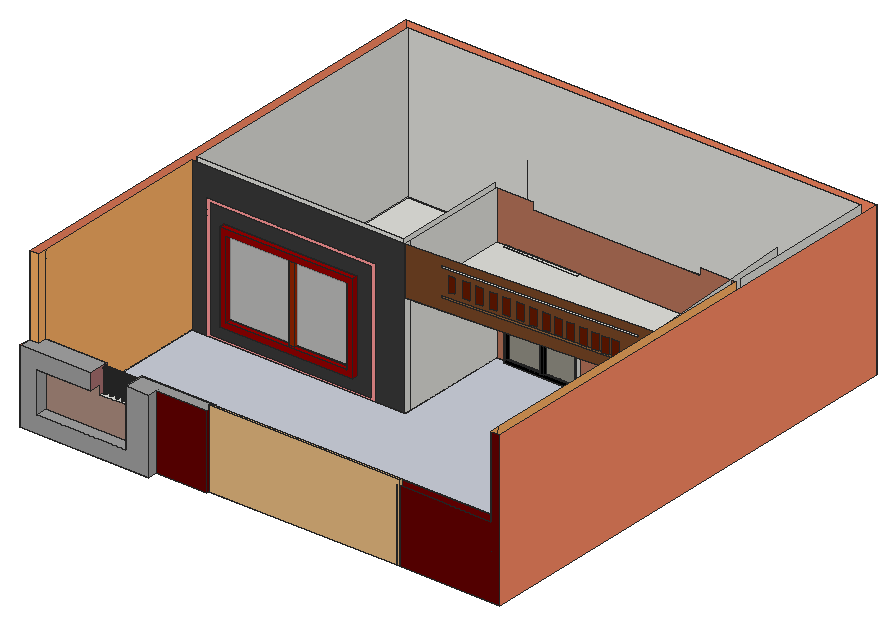
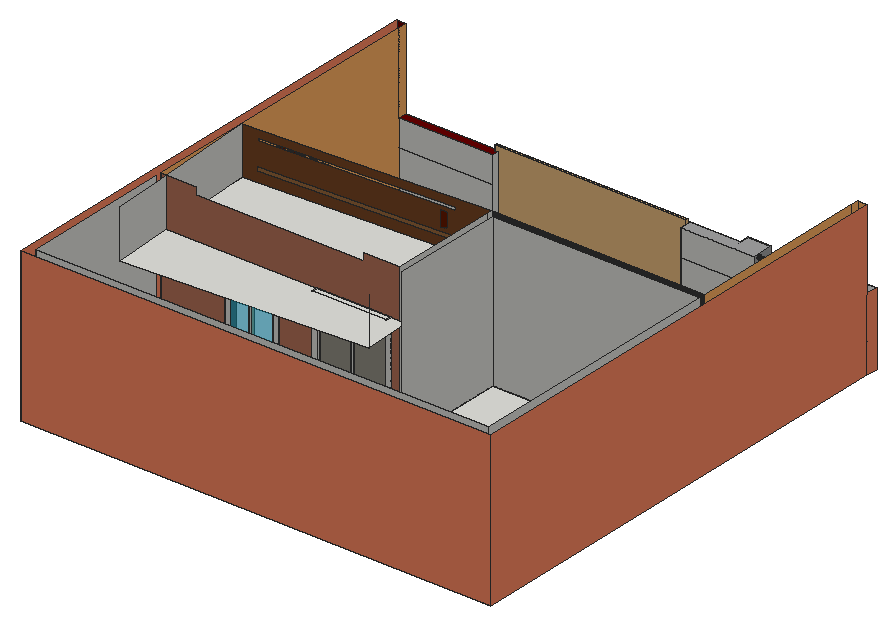
# SketchUp Ruby script. Lengths in inches.
U = 1.inch
M = Sketchup.active_model
def pt(a) = Geom::Point3d.new(a.map { |v| v * U })
def face(e, loops, mat)
  f = e.add_face(loops[0].map { |a| pt(a) })
  loops[1..].each { |l| e.add_face(l.map { |a| pt(a) }).erase! }
  f.material = f.back_material = mat if mat
  f
end
# faces: each face lists its corners as indices into pts; further lists are holes
def faces(e, pts, list, mat = nil) = list.each { |f| face(e, (f[0].is_a?(Array) ? f : [f]).map { |l| l.map { |i| pts[i] } }, mat) }
# xy, xz, yz: faces in a plane at the given z, y or x. An outline is a flat list of corners, or four numbers for a rectangle; further outlines are holes
def ring(l) = l.size == 4 ? [[l[0], l[1]], [l[2], l[1]], [l[2], l[3]], [l[0], l[3]]] : l.each_slice(2).to_a
def flat(e, list, mat, &to3) = list.each { |f| face(e, (f[0].is_a?(Array) ? f : [f]).map { |l| ring(l).map { |u, v| to3.(u, v) } }, mat) }
def xy(e, z, list, mat = nil) = flat(e, list, mat) { |x, y| [x, y, z] }
def xz(e, y, list, mat = nil) = flat(e, list, mat) { |x, z| [x, y, z] }
def yz(e, x, list, mat = nil) = flat(e, list, mat) { |y, z| [x, y, z] }
def lines(e, pts, list) = list.each { |a, b| e.add_line(pt(pts[a]), pt(pts[b])) }
# prism: a flat outline (further loops are holes) pulled along v
def prism(e, loops, v, mat = nil)
  f = face(e, loops, mat); d = Geom::Vector3d.new(v.map { |x| x * U })
  f.pushpull(f.normal.samedirection?(d) ? d.length : -d.length)
end
def box(e, o, s, mat = nil) = prism(e, [[o, [o[0] + s[0], o[1], o[2]], [o[0] + s[0], o[1] + s[1], o[2]], [o[0], o[1] + s[1], o[2]]]], [0, 0, s[2]], mat)
def at(x, y, z, deg = 0) = Geom::Transformation.translation(pt([x, y, z])) * Geom::Transformation.rotation(ORIGIN, Z_AXIS, deg.degrees)
def axes(o, x, y, z) = Geom::Transformation.new([*x, 0, *y, 0, *z, 0, *pt(o).to_a, 1])
def part(name) = M.definitions.add(name)
# library, detail: a bought-in or finely detailed component or shape, given as its bounding box
def library(name, o, s) = part(name).tap { |d| box(d.entities, o, s) }
def detail(e, o, s) = box(e.add_group.entities, o, s)
def put(e, d, t, mat = nil) = e.add_instance(d, t).tap { |i| i.material = mat if mat }
def group(e, t, mat = nil) = e.add_group.tap { |g| g.transformation = t; g.material = mat if mat }.entities
root = M.entities
M.materials.add("[Color A02]").color = [255, 153, 153]
M.materials.add("[Color A07]").color = [153, 0, 0]
M.materials.add("[Color A08]").color = [102, 0, 0]
M.materials.add("[Color B03]").color = [255, 140, 101]
M.materials.add("[Color B07]").color = [153, 38, 0]
M.materials.add("[Color B08]").color = [102, 25, 0]
M.materials.add("[Color C03]").color = [255, 178, 101]
M.materials.add("[Color M06]").color = [86, 86, 86]
M.materials.add("[Color M07]").color = [58, 58, 58]
M.materials.add("[Color M09]").color = [0, 0, 0]
M.materials.add("[Formica Beige]").color = [211, 187, 149]
M.materials.add("[Formica Graystone]").color = [149, 146, 135]
M.materials.add("[Formica Speckled Grey]").color = [94, 105, 111]
M.materials.add("[Marble Carrara Floor Tile]").color = [204, 208, 219]
M.materials.add("[Metal Rusted]").color = [184, 117, 91]
M.materials.add("[Pavers Flagstone Gray]").color = [162, 162, 162]
M.materials.add("[Pavers Herringbone Brick]").color = [172, 115, 115]
M.materials.add("[Pavers Modular Brick]").color = [175, 143, 129]
M.materials.add("[Translucent Glass Tinted]").color = [8, 201, 241]
M.materials["[Translucent Glass Tinted]"].alpha = 0.48
M.materials.add("[Translucent Resin Crush Gray]").color = [184, 184, 184]
M.materials["[Translucent Resin Crush Gray]"].alpha = 0.8
M.materials.add("[Wood Floor]").color = [155, 105, 61]
M.materials.add("[Wood Veneer 01]").color = [120, 70, 37]
c1 = library("Modern+Gate+1",[0,0,0],[118.11,1.97,78.74])
xy(root,0,[[1.5,7.75,132.625,19.75],[132.625,16.75,132.625,19.75,1.5,19.75,1.5,499.75,481.5,499.75,481.5,19.75,376.06,19.75,376.06,28.75,472.5,28.75,472.5,331.6875,313.15,331.6875,313.15,337.6875,472.5,337.6875,472.5,490.75,10.5,490.75,10.5,221.25,222.3125,221.25,222.3125,337.6875,237.6875,337.6875,237.6875,331.6875,228.3125,331.6875,228.3125,215.25,10.5,215.25,10.5,28.75,184.33,28.75,184.33,16.75],[10.5,28.75,10.5,215.25,228.3125,215.25,228.3125,331.6875,237.6875,331.6875,237.6875,337.6875,313.15,337.6875,313.15,331.6875,472.5,331.6875,472.5,28.75],[10.5,221.25,10.5,490.75,472.5,490.75,472.5,337.6875,222.3125,337.6875,222.3125,221.25]])
xy(root,1.0625,[[237.6875,328.6875,313.15,331.6875],[237.6875,331.6875,313.15,337.6875]])
xy(root,1.0625,[[10.5,28.75,472.5,28.75,472.5,331.6875,313.15,331.6875,313.15,328.6875,237.6875,328.6875,237.6875,331.6875,228.3125,331.6875,228.3125,215.25,10.5,215.25]],"[Marble Carrara Floor Tile]")
xy(root,1.125,[[10.5,221.25,222.3125,221.25,222.3125,337.6875,472.5,337.6875,472.5,490.75,10.5,490.75]])
xy(root,4.0625,[[275.42,328.6875,279.09,331.6875]])
xy(root,4.0625,[[240.6875,328.6875,275.42,331.6875],[279.09,328.6875,310.15,331.6875]],"[Color M09]")
xy(root,17.12,[[18.4,7.75,108.71,19.75]],"[Pavers Flagstone Gray]")
xy(root,17.84,[[43.625,209.25,179.38,215.25]],"[Color A07]")
xy(root,23.84,[[111.5,212.25,117.62,215.25]])
xy(root,23.84,[[49.625,209.25,173.38,209.25,173.38,215.25,117.62,215.25,117.62,212.25,111.5,212.25,111.5,215.25,49.625,215.25]],"[Color A07]")
xy(root,26.73,[[352.36,325.6875,407.17,331.6875]])
xy(root,32.73,[[379.77,328.6875,382.79,331.6875]])
xy(root,32.73,[[358.36,325.6875,401.17,325.6875,401.17,331.6875,382.79,331.6875,382.79,328.6875,379.77,328.6875,379.77,331.6875,358.36,331.6875]],"[Formica Speckled Grey]")
xy(root,49.75,[[[73.27,19.75,108.71,28.75],[75.43,22.84,74.98,22.89,74.55,23.0625,74.1875,23.33,73.9,23.69,73.72,24.11,73.65,24.5625,73.7,25.02,73.87,25.44,74.14,25.81,74.5,26.09,74.92,26.28,75.37,26.34,75.82,26.29,76.25,26.125,76.62,25.85,76.9,25.5,77.08,25.08,77.15,24.625,77.1,24.17,76.93,23.75,76.66,23.38,76.3,23.09,75.89,22.91],[81.31,22.84,80.85,22.89,80.43,23.0625,80.0625,23.33,79.78,23.69,79.6,24.11,79.53,24.5625,79.58,25.02,79.75,25.44,80.02,25.81,80.375,26.09,80.79,26.28,81.24,26.34,81.7,26.29,82.125,26.125,82.49,25.85,82.78,25.5,82.96,25.08,83.03,24.625,82.98,24.17,82.81,23.75,82.54,23.38,82.18,23.09,81.76,22.91],[87.31,22.84,86.85,22.89,86.43,23.0625,86.0625,23.33,85.78,23.69,85.6,24.11,85.53,24.5625,85.58,25.02,85.75,25.44,86.02,25.81,86.375,26.09,86.79,26.28,87.24,26.34,87.7,26.29,88.125,26.125,88.49,25.85,88.78,25.5,88.96,25.08,89.03,24.625,88.98,24.17,88.81,23.75,88.54,23.38,88.18,23.09,87.76,22.91],[93.39,22.91,92.9375,22.96,92.51,23.125,92.15,23.4,91.86,23.75,91.68,24.17,91.61,24.625,91.66,25.08,91.83,25.5,92.1,25.87,92.46,26.15,92.88,26.34,93.33,26.41,93.78,26.35,94.21,26.1875,94.58,25.92,94.86,25.56,95.04,25.14,95.11,24.6875,95.06,24.23,94.89,23.81,94.62,23.44,94.26,23.16,93.84,22.97],[99.52,22.91,99.0625,22.96,98.64,23.125,98.27,23.4,97.99,23.75,97.8,24.17,97.74,24.625,97.79,25.08,97.95,25.5,98.23,25.87,98.58,26.15,99,26.34,99.45,26.41,99.91,26.35,100.33,26.1875,100.7,25.92,100.99,25.56,101.17,25.14,101.24,24.6875,101.18,24.23,101.02,23.81,100.75,23.44,100.39,23.16,99.97,22.97],[106.08,22.91,105.625,22.96,105.2,23.125,104.83,23.4,104.55,23.75,104.37,24.17,104.3,24.625,104.35,25.08,104.52,25.5,104.79,25.87,105.15,26.15,105.56,26.34,106.02,26.41,106.47,26.35,106.9,26.1875,107.26,25.92,107.55,25.56,107.73,25.14,107.8,24.6875,107.75,24.23,107.58,23.81,107.31,23.44,106.95,23.16,106.53,22.97]],[87.31,22.84,86.85,22.89,86.43,23.0625,86.0625,23.33,85.78,23.69,85.6,24.11,85.53,24.5625,85.58,25.02,85.75,25.44,86.02,25.81,86.375,26.09,86.79,26.28,87.24,26.34,87.7,26.29,88.125,26.125,88.49,25.85,88.78,25.5,88.96,25.08,89.03,24.625,88.98,24.17,88.81,23.75,88.54,23.38,88.18,23.09,87.76,22.91],[93.39,22.91,92.9375,22.96,92.51,23.125,92.15,23.4,91.86,23.75,91.68,24.17,91.61,24.625,91.66,25.08,91.83,25.5,92.1,25.87,92.46,26.15,92.88,26.34,93.33,26.41,93.78,26.35,94.21,26.1875,94.58,25.92,94.86,25.56,95.04,25.14,95.11,24.6875,95.06,24.23,94.89,23.81,94.62,23.44,94.26,23.16,93.84,22.97]])
xy(root,58.43,[[18.4,7.75,73.27,19.75]],"[Pavers Flagstone Gray]")
xy(root,71.625,[[81.31,22.84,81.76,22.91,82.18,23.09,82.54,23.38,82.81,23.75,82.97,24.16,82.98,24.17,83.03,24.625,82.96,25.08,82.78,25.5,82.65,25.66,82.49,25.85,82.125,26.125,81.7,26.29,81.24,26.34,80.79,26.28,80.375,26.09,80.02,25.81,79.91,25.66,79.75,25.44,79.58,25.02,79.53,24.5625,79.59,24.16,79.6,24.11,79.78,23.69,80.0625,23.33,80.43,23.0625,80.85,22.89]])
xy(root,71.86,[[87.31,22.84,87.76,22.91,88.18,23.09,88.54,23.38,88.81,23.75,88.85,23.85,85.71,23.85,85.78,23.69,86.0625,23.33,86.43,23.0625,86.85,22.89],[93.39,22.91,93.84,22.97,94.26,23.16,94.62,23.44,94.89,23.81,94.91,23.85,91.82,23.85,91.86,23.75,92.15,23.4,92.51,23.125,92.9375,22.96],[106.08,22.91,106.53,22.97,106.95,23.16,107.31,23.44,107.58,23.81,107.6,23.85,104.51,23.85,104.55,23.75,104.83,23.4,105.2,23.125,105.625,22.96],[85.71,23.85,88.85,23.85,88.98,24.17,89.03,24.625,88.96,25.08,88.78,25.5,88.49,25.85,88.34,25.97,86.22,25.97,86.02,25.81,85.75,25.44,85.58,25.02,85.53,24.5625,85.6,24.11],[91.82,23.85,94.91,23.85,95.06,24.23,95.11,24.6875,95.04,25.14,94.86,25.56,94.58,25.92,94.5,25.97,92.22,25.97,92.1,25.87,91.83,25.5,91.66,25.08,91.61,24.625,91.68,24.17],
  [104.51,23.85,107.6,23.85,107.75,24.23,107.8,24.6875,107.73,25.14,107.55,25.56,107.26,25.92,107.19,25.97,104.91,25.97,104.79,25.87,104.52,25.5,104.35,25.08,104.3,24.625,104.37,24.17],[86.22,25.97,88.34,25.97,88.125,26.125,87.7,26.29,87.24,26.34,86.79,26.28,86.375,26.09],[92.22,25.97,92.46,26.15,92.88,26.34,93.33,26.41,93.78,26.35,94.21,26.1875,94.5,25.97],[104.91,25.97,107.19,25.97,106.9,26.1875,106.47,26.35,106.02,26.41,105.56,26.34,105.15,26.15]])
xy(root,71.9375,[[75.43,22.84,75.89,22.91,76.3,23.09,76.66,23.38,76.93,23.75,77.1,24.17,77.15,24.625,77.08,25.08,76.9,25.5,76.62,25.85,76.25,26.125,75.82,26.29,75.37,26.34,74.92,26.28,74.5,26.09,74.14,25.81,73.87,25.44,73.7,25.02,73.65,24.5625,73.72,24.11,73.9,23.69,74.1875,23.33,74.55,23.0625,74.98,22.89]])
xy(root,72.17,[[99.52,22.91,99.97,22.97,100.39,23.16,100.75,23.44,100.87,23.61,98.1,23.61,98.27,23.4,98.64,23.125,99.0625,22.96],[98.1,23.61,100.87,23.61,101.02,23.81,101.18,24.23,101.24,24.6875,101.17,25.14,100.99,25.56,100.7,25.92,100.33,26.1875,100.28,26.21,98.7,26.21,98.58,26.15,98.23,25.87,97.95,25.5,97.79,25.08,97.74,24.625,97.8,24.17,97.99,23.75],[98.7,26.21,100.28,26.21,99.91,26.35,99.45,26.41,99,26.34]])
xy(root,73.875,[[376.06,19.75,472.5,28.75]],"[Color A08]")
xy(root,74.8125,[[1.5,7.75,73.27,7.75,73.27,28.75,10.5,28.75,10.5,19.75,1.5,19.75],[108.71,7.75,132.625,7.75,132.625,16.75,184.33,16.75,184.33,28.75,108.71,28.75]],"[Pavers Flagstone Gray]")
xy(root,83.04,[[379.77,328.6875,382.79,331.6875]])
xy(root,83.04,[[358.36,325.6875,358.36,331.6875,379.77,331.6875,379.77,328.6875,382.79,328.6875,382.79,331.6875,401.17,331.6875,401.17,325.6875]],"[Formica Speckled Grey]")
xy(root,89.04,[[352.36,325.6875,407.17,331.6875]],"[Formica Speckled Grey]")
xy(root,103.33,[[111.5,212.25,117.62,215.25]])
xy(root,103.33,[[49.625,209.25,49.625,215.25,111.5,215.25,111.5,212.25,117.62,212.25,117.62,215.25,173.38,215.25,173.38,209.25]],"[Color A07]")
xy(root,104.07,[[275.42,328.6875,279.09,331.6875]])
xy(root,104.07,[[240.6875,328.6875,275.42,331.6875],[279.09,328.6875,310.15,331.6875]],"[Color M09]")
xy(root,107.07,[[[228.3125,215.25,219.69,382.03,463.88,394.65,472.5,227.87],[237.6875,328.6875,313.15,337.6875]],[237.6875,328.6875,313.15,331.6875],[237.6875,331.6875,313.15,337.6875]])
xy(root,109.33,[[43.625,209.25,179.38,215.25]],"[Color A07]")
xz(root,7.75,[[1.5,0,132.625,0,132.625,74.8125,108.71,74.8125,108.71,17.12,18.4,17.12,18.4,58.43,73.27,58.43,73.27,74.8125,1.5,74.8125]],"[Pavers Flagstone Gray]")
xz(root,16.75,[[132.625,0,184.33,74.8125]],"[Color A08]")
xz(root,19.75,[[376.06,0,481.5,0,481.5,156,472.5,156,472.5,73.875,376.06,73.875]],"[Color A08]")
xz(root,19.75,[[1.5,74.8125,10.5,156]],"[Color C03]")
xz(root,19.75,[[18.4,17.12,108.71,17.12,108.71,49.75,73.27,49.75,73.27,58.43,18.4,58.43]],"[Pavers Modular Brick]")
xz(root,28.75,[[10.5,0,184.33,1.0625],[184.33,0,376.06,1.0625],[376.06,0,472.5,1.0625],[10.5,1.0625,184.33,46.625],[376.06,1.0625,472.5,46.625],
  [10.5,46.625,10.5,74.8125,73.27,74.8125,73.27,49.75,108.71,49.75,108.71,74.8125,184.33,74.8125,184.33,46.625],[376.06,46.625,472.5,73.875]])
xz(root,209.25,[[[43.625,17.84,179.38,109.33],[49.625,23.84,173.38,103.33]]],"[Color A07]")
xz(root,212.25,[[111.5,23.84,117.62,103.33]],"[Color B07]")
xz(root,215.25,[[10.5,0,25.78,1.0625],[25.78,0,197.22,1.0625],[197.22,0,228.3125,1.0625],[[43.625,17.84,179.38,109.33],[49.625,23.84,173.38,103.33]],[111.5,23.84,117.62,103.33]])
xz(root,215.25,[[[25.78,1.0625,197.22,127.17],[28.54,2.76,194.46,124.41]]],"[Color A02]")
xz(root,215.25,[[10.5,1.0625,25.78,1.0625,25.78,127.17,197.22,127.17,197.22,1.0625,228.3125,1.0625,228.3125,156,10.5,156],[[28.54,2.76,194.46,124.41],[43.625,17.84,179.38,109.33]]],"[Color M07]")
xz(root,215.25,[[49.625,23.84,111.5,103.33],[117.62,23.84,173.38,103.33]],"[Translucent Resin Crush Gray]")
xz(root,221.25,[[10.5,0,222.3125,1.125],[10.5,1.125,222.3125,156]])
xz(root,325.6875,[[[352.36,26.73,407.17,89.04],[358.36,32.73,401.17,83.04]]],"[Formica Speckled Grey]")
xz(root,328.6875,[[[237.6875,1.0625,313.15,107.07],[240.6875,4.0625,310.15,104.07]],[275.42,4.0625,279.09,104.07]],"[Color M09]")
xz(root,328.6875,[[379.77,32.73,382.79,83.04]],"[Formica Beige]")
xz(root,331.6875,[[228.3125,0,237.6875,1.0625],[313.15,0,472.5,1.0625],[[237.6875,1.0625,313.15,107.07],[240.6875,4.0625,310.15,104.07]],[275.42,4.0625,279.09,104.07],[[352.36,26.73,407.17,89.04],[358.36,32.73,401.17,83.04]],
  [379.77,32.73,382.79,83.04]])
xz(root,331.6875,[[240.6875,4.0625,275.42,104.07],[279.09,4.0625,310.15,104.07]],"[Formica Graystone]")
xz(root,331.6875,[[[228.3125,1.0625,237.6875,1.0625,237.6875,107.07,313.15,107.07,313.15,1.0625,472.5,1.0625,472.5,156,437.11,156,437.11,149,265.66,149,265.66,156,228.3125,156],[352.36,26.73,407.17,89.04]]],"[Metal Rusted]")
xz(root,331.6875,[[358.36,32.73,379.77,83.04],[382.79,32.73,401.17,83.04]],"[Translucent Glass Tinted]")
xz(root,337.6875,[[222.3125,0,237.6875,1.125],[237.6875,0,313.15,1.0625],[313.15,0,472.5,1.125],[237.6875,1.0625,313.15,1.125]])
xz(root,490.75,[[10.5,0,472.5,1.125],[10.5,1.125,472.5,156]])
xz(root,499.75,[[1.5,0,481.5,156]],"[Color B03]")
yz(root,1.5,[[7.75,0,19.75,74.8125],[19.75,0,499.75,156]],"[Color B03]")
yz(root,10.5,[[28.75,0,215.25,1.0625],[221.25,0,490.75,1.125],[221.25,1.125,490.75,156]])
yz(root,10.5,[[28.75,1.0625,215.25,156],[19.75,74.8125,28.75,156]],"[Color C03]")
yz(root,18.4,[[7.75,17.12,19.75,58.43]],"[Pavers Flagstone Gray]")
yz(root,43.625,[[209.25,17.84,215.25,109.33]],"[Color A07]")
yz(root,49.625,[[209.25,23.84,215.25,103.33]],"[Color A07]")
yz(root,73.27,[[[19.75,49.75,28.75,49.75,28.75,74.8125,7.75,74.8125,7.75,58.43,19.75,58.43],[24.91,71.42,24.52,71.47,24.16,71.625,23.85,71.86,23.61,72.17,23.46,72.54,23.41,72.92,23.46,73.3125,23.61,73.67,23.85,73.98,24.16,74.22,24.52,74.37,24.91,74.42,25.3,74.37,25.66,74.22,25.97,73.98,26.21,73.67,26.36,73.3125,26.41,72.92,26.36,72.54,26.21,72.17,25.97,71.86,25.66,71.625,25.3,71.47]]],"[Pavers Herringbone Brick]")
yz(root,108.71,[[7.75,17.12,19.75,49.75],[[7.75,49.75,28.75,74.8125],[24.91,71.42,25.3,71.47,25.66,71.625,25.97,71.86,26.21,72.17,26.36,72.54,26.41,72.92,26.36,73.3125,26.21,73.67,25.97,73.98,25.66,74.22,25.3,74.37,24.91,74.42,24.52,74.37,24.16,74.22,23.85,73.98,23.61,73.67,23.46,73.3125,23.41,72.92,23.46,72.54,23.61,72.17,23.85,71.86,24.16,71.625,24.52,71.47]]],"[Pavers Flagstone Gray]")
yz(root,111.5,[[212.25,23.84,215.25,103.33]],"[Color B07]")
yz(root,117.62,[[212.25,23.84,215.25,103.33]],"[Color B07]")
yz(root,132.625,[[7.75,0,16.75,74.8125]],"[Pavers Flagstone Gray]")
yz(root,173.38,[[209.25,23.84,215.25,103.33]],"[Color A07]")
yz(root,179.38,[[209.25,17.84,215.25,109.33]],"[Color A07]")
yz(root,184.33,[[16.75,0,28.75,74.8125]],"[Color A08]")
yz(root,222.3125,[[221.25,0,337.6875,1.125],[221.25,1.125,337.6875,156]])
yz(root,228.3125,[[215.25,0,221.25,1.0625],[221.25,0,331.6875,1.0625],[215.25,1.0625,221.25,156],[221.25,1.0625,331.6875,156]])
yz(root,237.6875,[[331.6875,0,337.6875,1.0625],[328.6875,1.0625,331.6875,107.07],[331.6875,1.0625,337.6875,107.07]])
yz(root,240.6875,[[328.6875,4.0625,331.6875,104.07]],"[Color M09]")
yz(root,275.42,[[328.6875,4.0625,331.6875,104.07]],"[Color M09]")
yz(root,279.09,[[328.6875,4.0625,331.6875,104.07]],"[Color M09]")
yz(root,310.15,[[328.6875,4.0625,331.6875,104.07]],"[Color M09]")
yz(root,313.15,[[331.6875,0,337.6875,1.0625],[328.6875,1.0625,331.6875,107.07],[331.6875,1.0625,337.6875,107.07]])
yz(root,352.36,[[325.6875,26.73,331.6875,89.04]],"[Formica Speckled Grey]")
yz(root,358.36,[[325.6875,32.73,331.6875,83.04]],"[Formica Speckled Grey]")
yz(root,376.06,[[19.75,0,28.75,73.875]])
yz(root,379.77,[[328.6875,32.73,331.6875,83.04]],"[Formica Beige]")
yz(root,382.79,[[328.6875,32.73,331.6875,83.04]],"[Formica Beige]")
yz(root,401.17,[[325.6875,32.73,331.6875,83.04]],"[Formica Speckled Grey]")
yz(root,407.17,[[325.6875,26.73,331.6875,89.04]],"[Formica Speckled Grey]")
yz(root,472.5,[[28.75,0,331.6875,1.0625],[337.6875,0,490.75,1.125],[337.6875,1.125,490.75,156]])
yz(root,472.5,[[28.75,1.0625,331.6875,156],[19.75,73.875,28.75,156]],"[Color C03]")
yz(root,481.5,[[19.75,0,499.75,156]],"[Color B03]")
p = [[74.98,22.89,49.75],[75.43,22.84,49.75],[75.43,22.84,71.9375],[74.98,22.89,71.9375],[75.89,22.91,49.75],[75.89,22.91,71.9375],
  [80.85,22.89,49.75],[81.31,22.84,49.75],[81.31,22.84,71.625],[80.85,22.89,71.625],[81.76,22.91,49.75],[81.76,22.91,71.625],
  [86.85,22.89,49.75],[87.31,22.84,49.75],[87.31,22.84,71.86],[86.85,22.89,71.86],[87.76,22.91,49.75],[87.76,22.91,71.86],
  [74.55,23.0625,49.75],[74.55,23.0625,71.9375],[76.3,23.09,49.75],[76.3,23.09,71.9375],[80.43,23.0625,49.75],[80.43,23.0625,71.625],
  [82.18,23.09,49.75],[82.18,23.09,71.625],[86.43,23.0625,49.75],[86.43,23.0625,71.86],[88.18,23.09,49.75],[88.18,23.09,71.86],
  [92.9375,22.96,49.75],[93.39,22.91,49.75],[93.39,22.91,71.86],[92.9375,22.96,71.86],[93.84,22.97,49.75],[93.84,22.97,71.86],
  [99.0625,22.96,49.75],[99.52,22.91,49.75],[99.52,22.91,72.17],[99.0625,22.96,72.17],[99.97,22.97,49.75],[99.97,22.97,72.17],
  [105.625,22.96,49.75],[106.08,22.91,49.75],[106.08,22.91,71.86],[105.625,22.96,71.86],[106.53,22.97,49.75],[106.53,22.97,71.86],
  [92.51,23.125,49.75],[92.51,23.125,71.86],[94.26,23.16,49.75],[94.26,23.16,71.86],[98.64,23.125,49.75],[98.64,23.125,72.17],
  [100.39,23.16,49.75],[100.39,23.16,72.17],[105.2,23.125,49.75],[105.2,23.125,71.86],[106.95,23.16,49.75],[106.95,23.16,71.86],
  [74.1875,23.33,49.75],[74.1875,23.33,71.9375],[76.66,23.38,49.75],[76.66,23.38,71.9375],[80.0625,23.33,49.75],[80.0625,23.33,71.625],
  [82.54,23.38,49.75],[82.54,23.38,71.625],[86.0625,23.33,49.75],[86.0625,23.33,71.86],[88.54,23.38,49.75],[88.54,23.38,71.86],
  [92.15,23.4,49.75],[92.15,23.4,71.86],[98.27,23.4,49.75],[98.27,23.4,72.17],[104.83,23.4,49.75],[104.83,23.4,71.86],
  [94.62,23.44,49.75],[94.62,23.44,71.86],[100.75,23.44,49.75],[100.75,23.44,72.17],[107.31,23.44,49.75],[107.31,23.44,71.86],
  [73.9,23.69,49.75],[73.9,23.69,71.9375],[79.78,23.69,49.75],[79.78,23.69,71.625],[85.78,23.69,49.75],[85.78,23.69,71.86],
  [76.93,23.75,49.75],[76.93,23.75,71.9375],[82.81,23.75,49.75],[82.81,23.75,71.625],[88.81,23.75,49.75],[88.81,23.75,71.86],
  [91.86,23.75,49.75],[91.86,23.75,71.86],[94.89,23.81,49.75],[94.89,23.81,71.86],[97.99,23.75,49.75],[98.1,23.61,72.17],
  [97.99,23.75,72.17],[101.02,23.81,49.75],[101.02,23.81,72.17],[100.87,23.61,72.17],[104.55,23.75,49.75],[104.55,23.75,71.86],
  [107.58,23.81,49.75],[107.58,23.81,71.86],[73.72,24.11,49.75],[73.72,24.11,71.9375],[77.1,24.17,49.75],[77.1,24.17,71.9375],
  [79.6,24.11,49.75],[79.6,24.11,71.625],[82.98,24.17,49.75],[82.98,24.17,71.625],[82.97,24.16,71.625],[85.6,24.11,49.75],
  [85.71,23.85,71.86],[85.6,24.11,71.86],[88.98,24.17,49.75],[88.98,24.17,71.86],[88.85,23.85,71.86],[91.68,24.17,49.75],
  [91.82,23.85,71.86],[91.68,24.17,71.86],[95.06,24.23,49.75],[95.06,24.23,71.86],[94.91,23.85,71.86],[97.8,24.17,49.75],
  [97.8,24.17,72.17],[101.18,24.23,49.75],[101.18,24.23,72.17],[104.37,24.17,49.75],[104.51,23.85,71.86],[104.37,24.17,71.86],
  [107.75,24.23,49.75],[107.75,24.23,71.86],[107.6,23.85,71.86],[73.65,24.5625,49.75],[73.65,24.5625,71.9375],[79.53,24.5625,49.75],
  [79.59,24.16,71.625],[79.53,24.5625,71.625],[85.53,24.5625,49.75],[85.53,24.5625,71.86],[77.15,24.625,49.75],[77.15,24.625,71.9375],
  [83.03,24.625,49.75],[83.03,24.625,71.625],[89.03,24.625,49.75],[89.03,24.625,71.86],[91.61,24.625,49.75],[91.61,24.625,71.86],
  [95.11,24.6875,49.75],[95.11,24.6875,71.86],[97.74,24.625,49.75],[97.74,24.625,72.17],[101.24,24.6875,49.75],[101.24,24.6875,72.17],
  [104.3,24.625,49.75],[104.3,24.625,71.86],[107.8,24.6875,49.75],[107.8,24.6875,71.86],[73.7,25.02,49.75],[73.7,25.02,71.9375],
  [77.08,25.08,49.75],[77.08,25.08,71.9375],[79.58,25.02,49.75],[79.58,25.02,71.625],[82.96,25.08,49.75],[82.96,25.08,71.625],
  [85.58,25.02,49.75],[85.58,25.02,71.86],[88.96,25.08,49.75],[88.96,25.08,71.86],[91.66,25.08,49.75],[91.66,25.08,71.86],
  [97.79,25.08,49.75],[97.79,25.08,72.17],[104.35,25.08,49.75],[104.35,25.08,71.86],[95.04,25.14,49.75],[95.04,25.14,71.86],
  [101.17,25.14,49.75],[101.17,25.14,72.17],[107.73,25.14,49.75],[107.73,25.14,71.86],[73.87,25.44,49.75],[73.87,25.44,71.9375],
  [79.75,25.44,49.75],[79.75,25.44,71.625],[85.75,25.44,49.75],[85.75,25.44,71.86],[76.9,25.5,49.75],[76.9,25.5,71.9375],
  [82.78,25.5,49.75],[82.78,25.5,71.625],[88.78,25.5,49.75],[88.78,25.5,71.86],[91.83,25.5,49.75],[91.83,25.5,71.86],
  [94.86,25.56,49.75],[94.86,25.56,71.86],[97.95,25.5,49.75],[97.95,25.5,72.17],[100.99,25.56,49.75],[100.99,25.56,72.17],
  [104.52,25.5,49.75],[104.52,25.5,71.86],[107.55,25.56,49.75],[107.55,25.56,71.86],[74.14,25.81,49.75],[74.14,25.81,71.9375],
  [80.02,25.81,49.75],[79.91,25.66,71.625],[80.02,25.81,71.625],[86.02,25.81,49.75],[86.02,25.81,71.86],[76.62,25.85,49.75],
  [76.62,25.85,71.9375],[82.49,25.85,49.75],[82.49,25.85,71.625],[82.65,25.66,71.625],[88.49,25.85,49.75],[88.49,25.85,71.86],
  [92.1,25.87,49.75],[92.1,25.87,71.86],[98.23,25.87,49.75],[98.23,25.87,72.17],[104.79,25.87,49.75],[104.79,25.87,71.86],
  [94.58,25.92,49.75],[94.58,25.92,71.86],[100.7,25.92,49.75],[100.7,25.92,72.17],[107.26,25.92,49.75],[107.26,25.92,71.86],
  [74.5,26.09,49.75],[74.5,26.09,71.9375],[80.375,26.09,49.75],[80.375,26.09,71.625],[86.375,26.09,49.75],[86.22,25.97,71.86],
  [86.375,26.09,71.86],[76.25,26.125,49.75],[76.25,26.125,71.9375],[82.125,26.125,49.75],[82.125,26.125,71.625],[88.125,26.125,49.75],
  [88.125,26.125,71.86],[88.34,25.97,71.86],[92.46,26.15,49.75],[92.22,25.97,71.86],[92.46,26.15,71.86],[94.21,26.1875,49.75],
  [94.21,26.1875,71.86],[94.5,25.97,71.86],[98.58,26.15,49.75],[98.58,26.15,72.17],[100.33,26.1875,49.75],[100.33,26.1875,72.17],
  [105.15,26.15,49.75],[104.91,25.97,71.86],[105.15,26.15,71.86],[106.9,26.1875,49.75],[106.9,26.1875,71.86],[107.19,25.97,71.86],
  [74.92,26.28,49.75],[74.92,26.28,71.9375],[75.82,26.29,49.75],[75.82,26.29,71.9375],[80.79,26.28,49.75],[80.79,26.28,71.625],
  [81.7,26.29,49.75],[81.7,26.29,71.625],[86.79,26.28,49.75],[86.79,26.28,71.86],[87.7,26.29,49.75],[87.7,26.29,71.86],
  [92.88,26.34,49.75],[92.88,26.34,71.86],[93.78,26.35,49.75],[93.78,26.35,71.86],[99,26.34,49.75],[98.7,26.21,72.17],
  [99,26.34,72.17],[99.91,26.35,49.75],[99.91,26.35,72.17],[100.28,26.21,72.17],[105.56,26.34,49.75],[105.56,26.34,71.86],
  [106.47,26.35,49.75],[106.47,26.35,71.86],[75.37,26.34,49.75],[75.37,26.34,71.9375],[81.24,26.34,49.75],[81.24,26.34,71.625],
  [87.24,26.34,49.75],[87.24,26.34,71.86],[93.33,26.41,49.75],[93.33,26.41,71.86],[99.45,26.41,49.75],[99.45,26.41,72.17],
  [106.02,26.41,49.75],[106.02,26.41,71.86],[73.27,24.52,71.47],[73.27,24.91,71.42],[108.71,24.91,71.42],[108.71,24.52,71.47],
  [73.27,25.3,71.47],[108.71,25.3,71.47],[73.27,24.16,71.625],[108.71,24.16,71.625],[73.27,25.66,71.625],[108.71,25.66,71.625],
  [73.27,23.85,71.86],[108.71,23.85,71.86],[73.27,25.97,71.86],[108.71,25.97,71.86],[73.27,23.61,72.17],[108.71,23.61,72.17],
  [73.27,26.21,72.17],[108.71,26.21,72.17],[73.27,23.46,72.54],[108.71,23.46,72.54],[73.27,26.36,72.54],[108.71,26.36,72.54],
  [73.27,23.41,72.92],[108.71,23.41,72.92],[73.27,26.41,72.92],[108.71,26.41,72.92],[73.27,23.46,73.3125],[108.71,23.46,73.3125],
  [73.27,26.36,73.3125],[108.71,26.36,73.3125],[73.27,23.61,73.67],[108.71,23.61,73.67],[73.27,26.21,73.67],[108.71,26.21,73.67],
  [73.27,23.85,73.98],[108.71,23.85,73.98],[73.27,25.97,73.98],[108.71,25.97,73.98],[73.27,24.16,74.22],[108.71,24.16,74.22],
  [73.27,25.66,74.22],[108.71,25.66,74.22],[73.27,24.52,74.37],[108.71,24.52,74.37],[73.27,25.3,74.37],[108.71,25.3,74.37],
  [73.27,24.91,74.42],[108.71,24.91,74.42],[228.3125,215.25,107.07],[472.5,227.87,107.07],[472.5,227.87,156],[228.3125,215.25,156],
  [457.11,227.08,121.06],[457.11,227.08,117.75],[262.87,217.04,117.75],[262.87,217.04,121.06],[262.87,217.04,145.06],[262.87,217.04,148.37],
  [457.11,227.08,148.37],[457.11,227.08,145.06],[278.18,217.83,141.24],[278.18,217.83,125.37],[271.31,217.47,125.37],[271.31,217.47,141.24],
  [467.13,331.6875,156],[463.88,394.65,107.07],[463.88,394.65,156],[466.82,337.6875,156],[291.99,217.83,125.37],[291.99,217.83,141.24],
  [285.12,217.47,141.24],[285.12,217.47,125.37],[305.8,217.83,125.37],[305.8,217.83,141.24],[298.94,217.47,141.24],[298.94,217.47,125.37],
  [319.61,217.83,125.37],[319.61,217.83,141.24],[312.75,217.47,141.24],[312.75,217.47,125.37],[333.43,217.83,125.37],[333.43,217.83,141.24],
  [326.56,217.47,141.24],[326.56,217.47,125.37],[347.24,217.83,125.37],[347.24,217.83,141.24],[340.37,217.47,141.24],[340.37,217.47,125.37],
  [361.05,217.83,125.37],[361.05,217.83,141.24],[354.19,217.47,141.24],[354.19,217.47,125.37],[373.61,217.83,125.37],[373.61,217.83,141.24],
  [366.75,217.47,141.24],[366.75,217.47,125.37],[386.18,217.83,125.37],[386.18,217.83,141.24],[379.31,217.47,141.24],[379.31,217.47,125.37],
  [398.74,217.83,125.37],[398.74,217.83,141.24],[391.87,217.47,141.24],[391.87,217.47,125.37],[411.3,217.83,125.37],[411.3,217.83,141.24],
  [404.44,217.47,141.24],[404.44,217.47,125.37],[423.86,217.83,125.37],[423.86,217.83,141.24],[417,217.47,141.24],[417,217.47,125.37],
  [434.18,217.83,125.37],[434.18,217.83,141.24],[427.31,217.47,141.24],[427.31,217.47,125.37],[444.49,217.83,125.37],[444.49,217.83,141.24],
  [437.62,217.47,141.24],[437.62,217.47,125.37],[219.69,382.03,107.07],[219.69,382.03,156],[10.5,28.75,46.625],[10.5,19.75,46.625],
  [132.625,19.75,74.8125],[132.625,19.75,0],[472.5,28.75,46.625],[472.5,19.75,46.625]]
faces(root,p,[[0,1,2,3],[1,4,5,2],[6,7,8,9],[7,10,11,8],[12,13,14,15],[13,16,17,14],[18,0,3,19],[4,20,21,5],
  [22,6,9,23],[10,24,25,11],[26,12,15,27],[16,28,29,17],[30,31,32,33],[31,34,35,32],[36,37,38,39],[37,40,41,38],
  [42,43,44,45],[43,46,47,44],[48,30,33,49],[34,50,51,35],[52,36,39,53],[40,54,55,41],[56,42,45,57],[46,58,59,47],
  [60,18,19,61],[20,62,63,21],[64,22,23,65],[24,66,67,25],[68,26,27,69],[28,70,71,29],[72,48,49,73],[74,52,53,75],
  [76,56,57,77],[50,78,79,51],[54,80,81,55],[58,82,83,59],[84,60,61,85],[86,64,65,87],[88,68,69,89],[62,90,91,63],
  [66,92,93,67],[70,94,95,71],[96,72,73,97],[78,98,99,79],[100,74,75,101,102],[80,103,104,105,81],[106,76,77,107],[82,108,109,83],
  [110,84,85,111],[90,112,113,91],[114,86,87,115],[92,116,117,118,93],[119,88,89,120,121],[94,122,123,124,95],[125,96,97,126,127],[98,128,129,130,99],
  [131,100,102,132],[103,133,134,104],[135,106,107,136,137],[108,138,139,140,109],[141,110,111,142],[143,114,115,144,145],[146,119,121,147],[112,148,149,113],
  [116,150,151,117],[122,152,153,123],[154,125,127,155],[128,156,157,129],[158,131,132,159],[133,160,161,134],[162,135,137,163],[138,164,165,139],
  [166,141,142,167],[148,168,169,149],[170,143,145,171],[150,172,173,151],[174,146,147,175],[152,176,177,153],[178,154,155,179],[180,158,159,181],
  [182,162,163,183],[156,184,185,157],[160,186,187,161],[164,188,189,165],[190,166,167,191],[192,170,171,193],[194,174,175,195],[168,196,197,169],
  [172,198,199,173],[176,200,201,177],[202,178,179,203],[184,204,205,185],[206,180,181,207],[186,208,209,187],[210,182,183,211],[188,212,213,189],
  [214,190,191,215],[216,192,193,217,218],[219,194,195,220],[196,221,222,197],[198,223,224,225,199],[200,226,227,201],[228,202,203,229],[230,206,207,231],
  [232,210,211,233],[204,234,235,205],[208,236,237,209],[212,238,239,213],[240,214,215,241],[242,216,218,243],[244,219,220,245,246],[221,247,248,222],
  [223,249,250,224],[226,251,252,253,227],[254,228,229,255,256],[234,257,258,259,235],[260,230,231,261],[236,262,263,237],[264,232,233,265,266],[238,267,268,269,239],
  [270,240,241,271],[247,272,273,248],[274,242,243,275],[249,276,277,250],[278,244,246,279],[251,280,281,252],[282,254,256,283],[257,284,285,258],
  [286,260,261,287,288],[262,289,290,291,263],[292,264,266,293],[267,294,295,268],[296,270,271,297],[272,296,297,273],[298,274,275,299],[276,298,299,277],
  [300,278,279,301],[280,300,301,281],[302,282,283,303],[304,286,288,305],[306,292,293,307],[284,302,303,285],[289,304,305,290],[294,306,307,295],
  [308,309,310,311],[309,312,313,310],[314,308,311,315,118,144],[312,316,217,225,317,313],[318,314,144,118,315,319,140,136,130,126,124,120],[316,320,245,253,255,259,265,269,321,317,225,217],[322,318,120,124,126,130,136,140,319,323,105,101],[320,324,287,291,325,321,269,265,259,255,253,245],
  [326,322,101,105,323,327],[324,328,329,325,291,287],[330,326,327,331],[328,332,333,329],[334,330,331,335],[332,336,337,333],[338,334,335,339],[336,340,341,337],
  [342,338,339,343],[340,344,345,341],[346,342,343,347],[344,348,349,345],[350,346,347,351],[348,352,353,349],[354,350,351,355],[352,354,355,353]],"[Color M06]")
faces(root,p,[[[356,357,358,359],[360,361,362,363],[364,365,366,367],[368,369,370,371]]],"[Wood Veneer 01]")
faces(root,p,[[372,358,357,373,374,375]])
faces(root,p,[[363,362,361,360]],"[Wood Floor]")
faces(root,p,[[369,368,371,370],[376,377,378,379],[380,381,382,383],[384,385,386,387],[388,389,390,391],[392,393,394,395],[396,397,398,399],[400,401,402,403],
  [404,405,406,407],[408,409,410,411],[412,413,414,415],[416,417,418,419],[420,421,422,423],[424,425,426,427]],"[Color B08]")
lines(root,p,[[428,429],[430,431],[432,433],[434,435]])
put(root,c1,axes([184.33,22.74,0],[1.65005,0,0],[0,-1.5208,0],[0,0,1.0032]))
